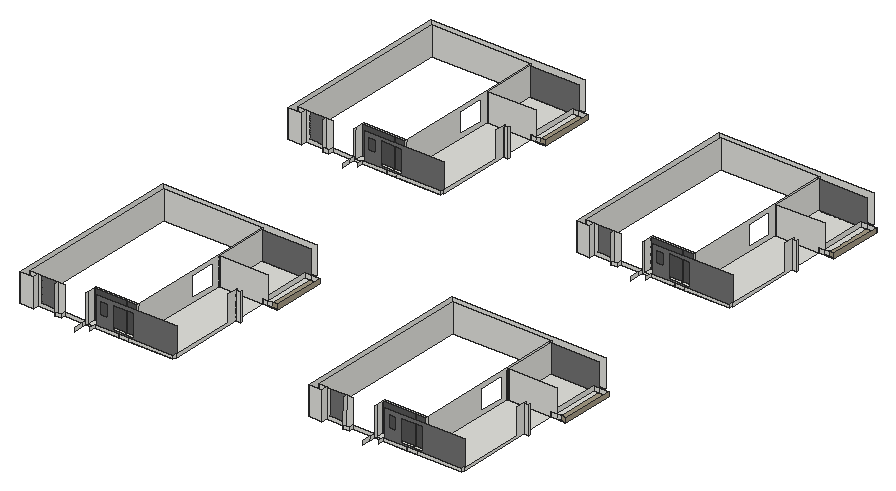
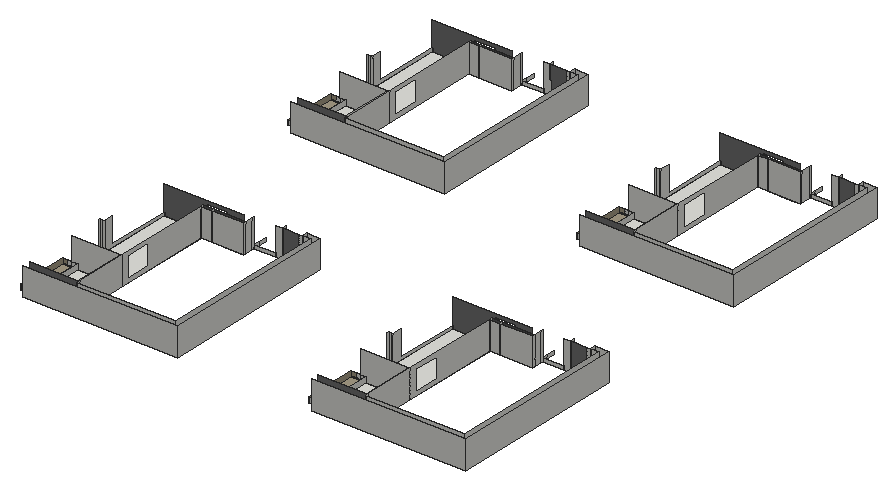
# SketchUp Ruby script. Lengths in inches.
U = 1.inch
M = Sketchup.active_model
def pt(a) = Geom::Point3d.new(a.map { |v| v * U })
def face(e, loops, mat)
  f = e.add_face(loops[0].map { |a| pt(a) })
  loops[1..].each { |l| e.add_face(l.map { |a| pt(a) }).erase! }
  f.material = f.back_material = mat if mat
  f
end
# faces: each face lists its corners as indices into pts; further lists are holes
def faces(e, pts, list, mat = nil) = list.each { |f| face(e, (f[0].is_a?(Array) ? f : [f]).map { |l| l.map { |i| pts[i] } }, mat) }
# xy, xz, yz: faces in a plane at the given z, y or x. An outline is a flat list of corners, or four numbers for a rectangle; further outlines are holes
def ring(l) = l.size == 4 ? [[l[0], l[1]], [l[2], l[1]], [l[2], l[3]], [l[0], l[3]]] : l.each_slice(2).to_a
def flat(e, list, mat, &to3) = list.each { |f| face(e, (f[0].is_a?(Array) ? f : [f]).map { |l| ring(l).map { |u, v| to3.(u, v) } }, mat) }
def xy(e, z, list, mat = nil) = flat(e, list, mat) { |x, y| [x, y, z] }
def xz(e, y, list, mat = nil) = flat(e, list, mat) { |x, z| [x, y, z] }
def yz(e, x, list, mat = nil) = flat(e, list, mat) { |y, z| [x, y, z] }
def lines(e, pts, list) = list.each { |a, b| e.add_line(pt(pts[a]), pt(pts[b])) }
# prism: a flat outline (further loops are holes) pulled along v
def prism(e, loops, v, mat = nil)
  f = face(e, loops, mat); d = Geom::Vector3d.new(v.map { |x| x * U })
  f.pushpull(f.normal.samedirection?(d) ? d.length : -d.length)
end
def box(e, o, s, mat = nil) = prism(e, [[o, [o[0] + s[0], o[1], o[2]], [o[0] + s[0], o[1] + s[1], o[2]], [o[0], o[1] + s[1], o[2]]]], [0, 0, s[2]], mat)
def at(x, y, z, deg = 0) = Geom::Transformation.translation(pt([x, y, z])) * Geom::Transformation.rotation(ORIGIN, Z_AXIS, deg.degrees)
def axes(o, x, y, z) = Geom::Transformation.new([*x, 0, *y, 0, *z, 0, *pt(o).to_a, 1])
def part(name) = M.definitions.add(name)
# library, detail: a bought-in or finely detailed component or shape, given as its bounding box
def library(name, o, s) = part(name).tap { |d| box(d.entities, o, s) }
def detail(e, o, s) = box(e.add_group.entities, o, s)
def put(e, d, t, mat = nil) = e.add_instance(d, t).tap { |i| i.material = mat if mat }
def group(e, t, mat = nil) = e.add_group.tap { |g| g.transformation = t; g.material = mat if mat }.entities
root = M.entities
M.materials.add("[Color M05]").color = [114, 114, 114]
M.materials.add("[Color M06]").color = [86, 86, 86]
M.materials.add("[Concrete Tile]").color = [165, 155, 133]
M.materials.add("[Granite Brown]").color = [89, 59, 61]
xy(root,1014,[[523.04,1822.9375,557.88,1833.75],[557.88,1822.9375,661.4375,1833.75],[661.4375,1822.9375,704.25,1835.1875],[704.25,1822.9375,890.875,1835.1875],[1741.23,1822.9375,1776.07,1833.75],
  [1776.07,1822.9375,1879.625,1833.75],[1879.625,1822.9375,1922.4375,1835.1875],[1922.4375,1822.9375,2109.0625,1835.1875],[523.04,1833.75,523.04,1865.75,557.4,1865.75,557.4,1835.1875,557.88,1835.1875,557.88,1833.75],[557.88,1833.75,661.4375,1835.1875],
  [1741.23,1833.75,1741.23,1865.75,1775.59,1865.75,1775.59,1835.1875,1776.07,1835.1875,1776.07,1833.75],[1776.07,1833.75,1879.625,1835.1875],[557.4,1835.1875,661.4375,1865.75],[661.4375,1835.1875,704.25,1865.75],[704.25,1835.1875,890.875,2295.875],
  [1775.59,1835.1875,1879.625,1865.75],[1879.625,1835.1875,1922.4375,1865.75],[1922.4375,1835.1875,2109.0625,2295.875],[523.04,1865.75,557.4,1876.125],[557.4,1865.75,661.4375,1876.125],
  [661.4375,1865.75,704.25,1876.125],[1741.23,1865.75,1775.59,1876.125],[1775.59,1865.75,1879.625,1876.125],[1879.625,1865.75,1922.4375,1876.125],[894.3125,2148.83,913.875,2156.01],
  [2112.5,2148.83,2132.0625,2156.01],[704.25,2295.875,710.125,2518.89],[710.125,2295.875,890.875,2518.89],[890.875,2295.875,913.875,2518.89],[1922.4375,2295.875,1928.3125,2518.89],
  [1928.3125,2295.875,2109.0625,2518.89],[2109.0625,2295.875,2132.0625,2518.89],[704.25,2518.89,890.875,2531.375],[1922.4375,2518.89,2109.0625,2531.375],[523.04,3237.625,557.88,3248.4375],
  [557.88,3237.625,661.4375,3248.4375],[661.4375,3237.625,704.25,3249.875],[704.25,3237.625,890.875,3249.875],[1741.23,3237.625,1776.07,3248.4375],[1776.07,3237.625,1879.625,3248.4375],
  [1879.625,3237.625,1922.4375,3249.875],[1922.4375,3237.625,2109.0625,3249.875],[523.04,3248.4375,523.04,3280.4375,557.4,3280.4375,557.4,3249.875,557.88,3249.875,557.88,3248.4375],[557.88,3248.4375,661.4375,3249.875],[1741.23,3248.4375,1741.23,3280.4375,1775.59,3280.4375,1775.59,3249.875,1776.07,3249.875,1776.07,3248.4375],
  [1776.07,3248.4375,1879.625,3249.875],[557.4,3249.875,661.4375,3280.4375],[661.4375,3249.875,704.25,3280.4375],[704.25,3249.875,890.875,3710.5625],[1775.59,3249.875,1879.625,3280.4375],
  [1879.625,3249.875,1922.4375,3280.4375],[1922.4375,3249.875,2109.0625,3710.5625],[523.04,3280.4375,557.4,3290.8125],[557.4,3280.4375,661.4375,3290.8125],[661.4375,3280.4375,704.25,3290.8125],
  [1741.23,3280.4375,1775.59,3290.8125],[1775.59,3280.4375,1879.625,3290.8125],[1879.625,3280.4375,1922.4375,3290.8125],[894.3125,3563.51,913.875,3570.7],[2112.5,3563.51,2132.0625,3570.7],
  [704.25,3710.5625,710.125,3933.57],[710.125,3710.5625,890.875,3933.57],[890.875,3710.5625,913.875,3933.57],[1922.4375,3710.5625,1928.3125,3933.57],[1928.3125,3710.5625,2109.0625,3933.57],
  [2109.0625,3710.5625,2132.0625,3933.57],[704.25,3933.57,890.875,3946.0625],[1922.4375,3933.57,2109.0625,3946.0625]])
xy(root,1014,[[913.875,2295.875,954.6875,2518.89],[2132.0625,2295.875,2172.875,2518.89],[913.875,3710.5625,954.6875,3933.57],[2132.0625,3710.5625,2172.875,3933.57]],"[Concrete Tile]")
xz(root,1799.9375,[[262.875,1014,319.53,1134],[1481.0625,1014,1537.72,1134]])
xz(root,1799.9375,[[557.4,1014,557.88,1026.6875],[1775.59,1014,1776.07,1026.6875]],"[Granite Brown]")
xz(root,1806.5625,[[403.69,1014,403.69,1029.4375,403.77,1029.4375],[403.69,1014,431.33,1014,431.33,1029.4375,403.77,1029.4375],[1621.88,1014,1621.88,1029.4375,1621.96,1029.4375],[1621.88,1014,1649.52,1014,1649.52,1029.4375,1621.96,1029.4375]])
xz(root,1822.9375,[[285.875,1014,319.53,1134],[319.53,1014,403.69,1014,403.69,1029.4375,334.58,1029.4375,334.58,1134,319.53,1134],[403.69,1014,404.29,1134,431.33,1134,431.33,1014],[431.33,1014,523.04,1029.4375],[557.88,1014,661.4375,1026.6875],
  [661.4375,1014,704.25,1026.6875],[704.25,1014,890.875,1026.6875],[1504.0625,1014,1537.72,1134],[1537.72,1014,1621.88,1014,1621.88,1029.4375,1552.77,1029.4375,1552.77,1134,1537.72,1134],[1621.88,1014,1622.48,1134,1649.52,1134,1649.52,1014],
  [1649.52,1014,1741.23,1029.4375],[1776.07,1014,1879.625,1026.6875],[1879.625,1014,1922.4375,1026.6875],[1922.4375,1014,2109.0625,1026.6875]])
xz(root,1822.9375,[[403.69,1014,404.29,1134,334.58,1134,334.58,1029.4375,403.69,1029.4375],[1621.88,1014,1622.48,1134,1552.77,1134,1552.77,1029.4375,1621.88,1029.4375]],"[Color M05]")
xz(root,1822.9375,[[557.4,1014,557.88,1026.6875],[1775.59,1014,1776.07,1026.6875]],"[Granite Brown]")
xz(root,1835.1875,[[890.875,1014,894.3125,1026.6875],[2109.0625,1014,2112.5,1026.6875]])
xz(root,1835.1875,[[[557.88,1014,890.875,1014,890.875,1026.6875,894.3125,1026.6875,894.3125,1134,557.88,1134],[646.53,1023.2,646.53,1023.51,625.7,1023.51,625.7,1121.33,715.63,1121.33,715.63,1023.2],[571.45,1064.45,603.76,1116.73]],[[1776.07,1014,2109.0625,1014,2109.0625,1026.6875,2112.5,1026.6875,2112.5,1134,1776.07,1134],[1864.72,1023.2,1864.72,1023.51,1843.88,1023.51,1843.88,1121.33,1933.82,1121.33,1933.82,1023.2],[1789.64,1064.45,1821.95,1116.73]]],"[Color M05]")
xz(root,1865.75,[[523.04,1014,661.4375,1134],[661.4375,1014,704.25,1134],[1741.23,1014,1879.625,1134],[1879.625,1014,1922.4375,1134]],"[Color M06]")
xz(root,1876.125,[[523.04,1014,661.4375,1134],[661.4375,1014,704.25,1134],[1741.23,1014,1879.625,1134],[1879.625,1014,1922.4375,1134]])
xz(root,2148.83,[[894.3125,1014,913.875,1134],[2112.5,1014,2132.0625,1134]])
xz(root,2156.01,[[894.3125,1014,913.875,1031.36],[2112.5,1014,2132.0625,1031.36]])
xz(root,2295.875,[[704.25,1014,710.125,1134],[710.125,1014,710.125,1134,913.875,1134,913.875,1034.8125,890.875,1034.8125,890.875,1014],[890.875,1014,913.875,1034.8125],[913.875,1014,930.75,1015.75],[930.75,1014,954.6875,1015.75],
  [1922.4375,1014,1928.3125,1134],[1928.3125,1014,1928.3125,1134,2132.0625,1134,2132.0625,1034.8125,2109.0625,1034.8125,2109.0625,1014],[2109.0625,1014,2132.0625,1034.8125],[2132.0625,1014,2148.9375,1015.75],[2148.9375,1014,2172.875,1015.75],
  [913.875,1015.75,930.75,1034.8125],[2132.0625,1015.75,2148.9375,1034.8125]])
xz(root,2295.875,[[930.75,1015.75,954.6875,1034.8125],[2148.9375,1015.75,2172.875,1034.8125]],"[Concrete Tile]")
xz(root,2518.89,[[704.25,1014,710.125,1134],[890.875,1014,913.875,1034.8125],[913.875,1014,954.6875,1034.8125],[1922.4375,1014,1928.3125,1134],[2109.0625,1014,2132.0625,1034.8125],
  [2132.0625,1014,2172.875,1034.8125]])
xz(root,2518.89,[[710.125,1014,890.875,1014,890.875,1034.8125,913.875,1034.8125,913.875,1134,710.125,1134],[1928.3125,1014,2109.0625,1014,2109.0625,1034.8125,2132.0625,1034.8125,2132.0625,1134,1928.3125,1134]],"[Color M05]")
xz(root,2531.375,[[285.875,1014,704.25,1134],[1504.0625,1014,1922.4375,1134]])
xz(root,2554.375,[[262.875,1014,913.875,1134],[1481.0625,1014,2132.0625,1134]])
xz(root,3214.625,[[262.875,1014,319.53,1134],[1481.0625,1014,1537.72,1134]])
xz(root,3214.625,[[557.4,1014,557.88,1026.6875],[1775.59,1014,1776.07,1026.6875]],"[Granite Brown]")
xz(root,3221.25,[[403.69,1014,403.69,1029.4375,403.77,1029.4375],[403.69,1014,431.33,1014,431.33,1029.4375,403.77,1029.4375],[1621.88,1014,1621.88,1029.4375,1621.96,1029.4375],[1621.88,1014,1649.52,1014,1649.52,1029.4375,1621.96,1029.4375]])
xz(root,3237.625,[[285.875,1014,319.53,1134],[319.53,1014,403.69,1014,403.69,1029.4375,334.58,1029.4375,334.58,1134,319.53,1134],[403.69,1014,404.29,1134,431.33,1134,431.33,1014],[431.33,1014,523.04,1029.4375],[557.88,1014,661.4375,1026.6875],
  [661.4375,1014,704.25,1026.6875],[704.25,1014,890.875,1026.6875],[1504.0625,1014,1537.72,1134],[1537.72,1014,1621.88,1014,1621.88,1029.4375,1552.77,1029.4375,1552.77,1134,1537.72,1134],[1621.88,1014,1622.48,1134,1649.52,1134,1649.52,1014],
  [1649.52,1014,1741.23,1029.4375],[1776.07,1014,1879.625,1026.6875],[1879.625,1014,1922.4375,1026.6875],[1922.4375,1014,2109.0625,1026.6875]])
xz(root,3237.625,[[403.69,1014,404.29,1134,334.58,1134,334.58,1029.4375,403.69,1029.4375],[1621.88,1014,1622.48,1134,1552.77,1134,1552.77,1029.4375,1621.88,1029.4375]],"[Color M05]")
xz(root,3237.625,[[557.4,1014,557.88,1026.6875],[1775.59,1014,1776.07,1026.6875]],"[Granite Brown]")
xz(root,3249.875,[[890.875,1014,894.3125,1026.6875],[2109.0625,1014,2112.5,1026.6875]])
xz(root,3249.875,[[[557.88,1014,890.875,1014,890.875,1026.6875,894.3125,1026.6875,894.3125,1134,557.88,1134],[646.53,1023.2,646.53,1023.51,625.7,1023.51,625.7,1121.33,715.63,1121.33,715.63,1023.2],[571.45,1064.45,603.76,1116.73]],[[1776.07,1014,2109.0625,1014,2109.0625,1026.6875,2112.5,1026.6875,2112.5,1134,1776.07,1134],[1864.72,1023.2,1864.72,1023.51,1843.88,1023.51,1843.88,1121.33,1933.82,1121.33,1933.82,1023.2],[1789.64,1064.45,1821.95,1116.73]]],"[Color M05]")
xz(root,3280.4375,[[523.04,1014,661.4375,1134],[661.4375,1014,704.25,1134],[1741.23,1014,1879.625,1134],[1879.625,1014,1922.4375,1134]],"[Color M06]")
xz(root,3290.8125,[[523.04,1014,661.4375,1134],[661.4375,1014,704.25,1134],[1741.23,1014,1879.625,1134],[1879.625,1014,1922.4375,1134]])
xz(root,3563.51,[[894.3125,1014,913.875,1134],[2112.5,1014,2132.0625,1134]])
xz(root,3570.7,[[894.3125,1014,913.875,1031.36],[2112.5,1014,2132.0625,1031.36]])
xz(root,3710.5625,[[704.25,1014,710.125,1134],[710.125,1014,710.125,1134,913.875,1134,913.875,1034.8125,890.875,1034.8125,890.875,1014],[890.875,1014,913.875,1034.8125],[913.875,1014,930.75,1015.75],[930.75,1014,954.6875,1015.75],
  [1922.4375,1014,1928.3125,1134],[1928.3125,1014,1928.3125,1134,2132.0625,1134,2132.0625,1034.8125,2109.0625,1034.8125,2109.0625,1014],[2109.0625,1014,2132.0625,1034.8125],[2132.0625,1014,2148.9375,1015.75],[2148.9375,1014,2172.875,1015.75],
  [913.875,1015.75,930.75,1034.8125],[2132.0625,1015.75,2148.9375,1034.8125]])
xz(root,3710.5625,[[930.75,1015.75,954.6875,1034.8125],[2148.9375,1015.75,2172.875,1034.8125]],"[Concrete Tile]")
xz(root,3933.57,[[704.25,1014,710.125,1134],[890.875,1014,913.875,1034.8125],[913.875,1014,954.6875,1034.8125],[1922.4375,1014,1928.3125,1134],[2109.0625,1014,2132.0625,1034.8125],
  [2132.0625,1014,2172.875,1034.8125]])
xz(root,3933.57,[[710.125,1014,890.875,1014,890.875,1034.8125,913.875,1034.8125,913.875,1134,710.125,1134],[1928.3125,1014,2109.0625,1014,2109.0625,1034.8125,2132.0625,1034.8125,2132.0625,1134,1928.3125,1134]],"[Color M05]")
xz(root,3946.0625,[[285.875,1014,704.25,1134],[1504.0625,1014,1922.4375,1134]])
xz(root,3969.0625,[[262.875,1014,913.875,1134],[1481.0625,1014,2132.0625,1134]])
yz(root,262.875,[[1799.9375,1014,2554.375,1134],[3214.625,1014,3969.0625,1134]])
yz(root,285.875,[[1822.9375,1014,2531.375,1134],[3237.625,1014,3946.0625,1134]])
yz(root,319.53,[[1799.9375,1014,1822.9375,1134],[3214.625,1014,3237.625,1134]])
yz(root,403.69,[[1806.5625,1014,1822.9375,1029.4375],[3221.25,1014,3237.625,1029.4375]])
yz(root,431.33,[[1806.5625,1014,1822.9375,1029.4375],[3221.25,1014,3237.625,1029.4375]])
yz(root,523.04,[[1763.25,1014,1799.9375,1029.4375],[1799.9375,1014,1822.9375,1029.4375],[1822.9375,1014,1833.75,1134],[1833.75,1014,1865.75,1134],[1865.75,1014,1876.125,1134],
  [3177.9375,1014,3214.625,1029.4375],[3214.625,1014,3237.625,1029.4375],[3237.625,1014,3248.4375,1134],[3248.4375,1014,3280.4375,1134],[3280.4375,1014,3290.8125,1134]])
yz(root,557.4,[[1799.9375,1014,1822.9375,1026.6875],[3214.625,1014,3237.625,1026.6875]])
yz(root,661.4375,[[1822.9375,1014,1833.75,1026.6875],[1865.75,1014,1876.125,1134],[3237.625,1014,3248.4375,1026.6875],[3280.4375,1014,3290.8125,1134]])
yz(root,704.25,[[1865.75,1014,1876.125,1134],[[1876.125,1014,2295.875,1134],[2156.01,1031.36,2266.33,1117.04]],[2295.875,1014,2518.89,1134],[2518.89,1014,2531.375,1134],[3280.4375,1014,3290.8125,1134],
  [[3290.8125,1014,3710.5625,1134],[3570.7,1031.36,3681.01,1117.04]],[3710.5625,1014,3933.57,1134],[3933.57,1014,3946.0625,1134]])
yz(root,710.125,[[2295.875,1014,2518.89,1134],[3710.5625,1014,3933.57,1134]])
yz(root,890.875,[[1822.9375,1014,1835.1875,1026.6875],[2295.875,1014,2518.89,1034.8125],[3237.625,1014,3249.875,1026.6875],[3710.5625,1014,3933.57,1034.8125]])
yz(root,894.3125,[[1835.1875,1014,2148.83,1014,2148.83,1134,2108.8,1134,2108.8,1026.6875,1835.1875,1026.6875],[2148.83,1014,2156.01,1134],[3249.875,1014,3563.51,1014,3563.51,1134,3523.49,1134,3523.49,1026.6875,3249.875,1026.6875],[3563.51,1014,3570.7,1134]])
yz(root,913.875,[[2148.83,1014,2156.01,1134],[3563.51,1014,3570.7,1134]])
yz(root,954.6875,[[2295.875,1014,2518.89,1034.8125],[3710.5625,1014,3933.57,1034.8125]],"[Concrete Tile]")
yz(root,1481.0625,[[1799.9375,1014,2554.375,1134],[3214.625,1014,3969.0625,1134]])
yz(root,1504.0625,[[1822.9375,1014,2531.375,1134],[3237.625,1014,3946.0625,1134]])
yz(root,1537.72,[[1799.9375,1014,1822.9375,1134],[3214.625,1014,3237.625,1134]])
yz(root,1621.88,[[1806.5625,1014,1822.9375,1029.4375],[3221.25,1014,3237.625,1029.4375]])
yz(root,1649.52,[[1806.5625,1014,1822.9375,1029.4375],[3221.25,1014,3237.625,1029.4375]])
yz(root,1741.23,[[1763.25,1014,1799.9375,1029.4375],[1799.9375,1014,1822.9375,1029.4375],[1822.9375,1014,1833.75,1134],[1833.75,1014,1865.75,1134],[1865.75,1014,1876.125,1134],
  [3177.9375,1014,3214.625,1029.4375],[3214.625,1014,3237.625,1029.4375],[3237.625,1014,3248.4375,1134],[3248.4375,1014,3280.4375,1134],[3280.4375,1014,3290.8125,1134]])
yz(root,1775.59,[[1799.9375,1014,1822.9375,1026.6875],[3214.625,1014,3237.625,1026.6875]])
yz(root,1879.625,[[1822.9375,1014,1833.75,1026.6875],[1865.75,1014,1876.125,1134],[3237.625,1014,3248.4375,1026.6875],[3280.4375,1014,3290.8125,1134]])
yz(root,1922.4375,[[1865.75,1014,1876.125,1134],[[1876.125,1014,2295.875,1134],[2156.01,1031.36,2266.33,1117.04]],[2295.875,1014,2518.89,1134],[2518.89,1014,2531.375,1134],[3280.4375,1014,3290.8125,1134],
  [[3290.8125,1014,3710.5625,1134],[3570.7,1031.36,3681.01,1117.04]],[3710.5625,1014,3933.57,1134],[3933.57,1014,3946.0625,1134]])
yz(root,1928.3125,[[2295.875,1014,2518.89,1134],[3710.5625,1014,3933.57,1134]])
yz(root,2109.0625,[[1822.9375,1014,1835.1875,1026.6875],[2295.875,1014,2518.89,1034.8125],[3237.625,1014,3249.875,1026.6875],[3710.5625,1014,3933.57,1034.8125]])
yz(root,2112.5,[[1835.1875,1014,2148.83,1014,2148.83,1134,2108.8,1134,2108.8,1026.6875,1835.1875,1026.6875],[2148.83,1014,2156.01,1134],[3249.875,1014,3563.51,1014,3563.51,1134,3523.49,1134,3523.49,1026.6875,3249.875,1026.6875],[3563.51,1014,3570.7,1134]])
yz(root,2132.0625,[[2148.83,1014,2156.01,1134],[3563.51,1014,3570.7,1134]])
yz(root,2172.875,[[2295.875,1014,2518.89,1034.8125],[3710.5625,1014,3933.57,1034.8125]],"[Concrete Tile]")
p = [[403.69,1822.9375,1014],[403.69,1806.5625,1014],[403.77,1806.5625,1029.4375],[404.29,1806.5625,1134],[404.29,1822.9375,1134],[1621.88,1822.9375,1014],
  [1621.88,1806.5625,1014],[1621.96,1806.5625,1029.4375],[1622.48,1806.5625,1134],[1622.48,1822.9375,1134],[403.69,3237.625,1014],[403.69,3221.25,1014],
  [403.77,3221.25,1029.4375],[404.29,3221.25,1134],[404.29,3237.625,1134],[1621.88,3237.625,1014],[1621.88,3221.25,1014],[1621.96,3221.25,1029.4375],
  [1622.48,3221.25,1134],[1622.48,3237.625,1134]]
faces(root,p,[[0,1,2,3,4],[5,6,7,8,9],[10,11,12,13,14],[15,16,17,18,19]])
